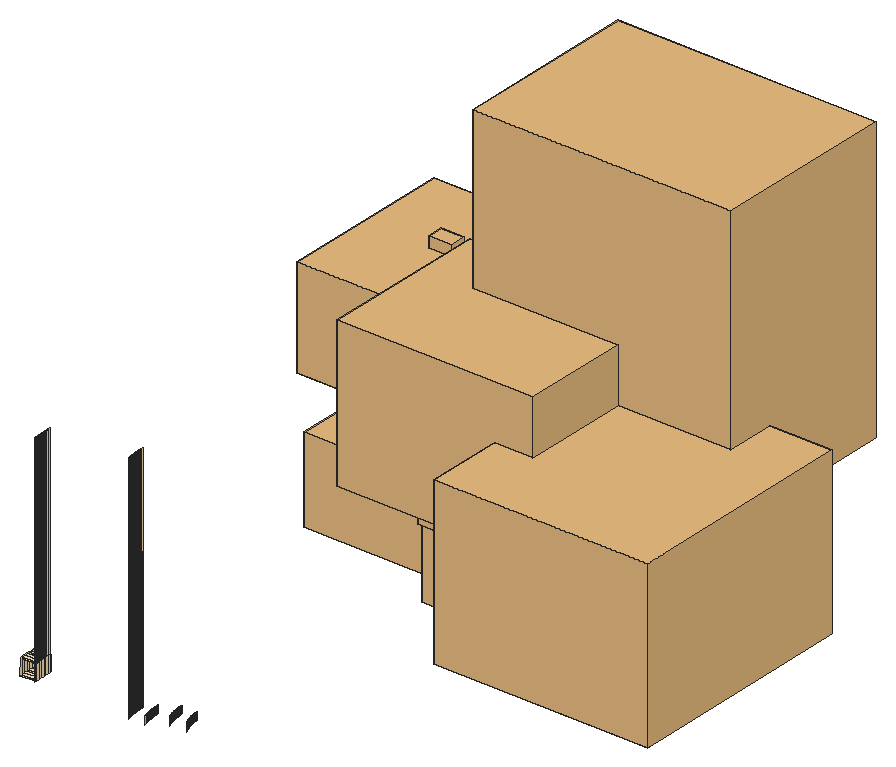
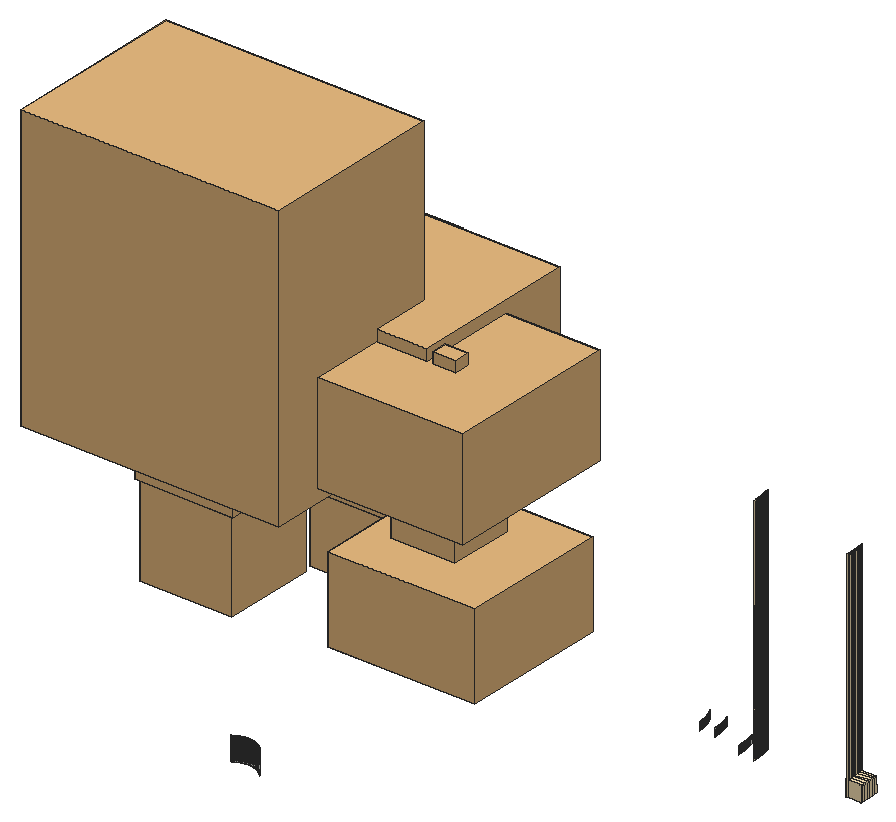
# SketchUp Ruby script. Lengths in inches.
U = 1.inch
M = Sketchup.active_model
def pt(a) = Geom::Point3d.new(a.map { |v| v * U })
def face(e, loops, mat)
  f = e.add_face(loops[0].map { |a| pt(a) })
  loops[1..].each { |l| e.add_face(l.map { |a| pt(a) }).erase! }
  f.material = f.back_material = mat if mat
  f
end
# faces: each face lists its corners as indices into pts; further lists are holes
def faces(e, pts, list, mat = nil) = list.each { |f| face(e, (f[0].is_a?(Array) ? f : [f]).map { |l| l.map { |i| pts[i] } }, mat) }
# xy, xz, yz: faces in a plane at the given z, y or x. An outline is a flat list of corners, or four numbers for a rectangle; further outlines are holes
def ring(l) = l.size == 4 ? [[l[0], l[1]], [l[2], l[1]], [l[2], l[3]], [l[0], l[3]]] : l.each_slice(2).to_a
def flat(e, list, mat, &to3) = list.each { |f| face(e, (f[0].is_a?(Array) ? f : [f]).map { |l| ring(l).map { |u, v| to3.(u, v) } }, mat) }
def xy(e, z, list, mat = nil) = flat(e, list, mat) { |x, y| [x, y, z] }
def xz(e, y, list, mat = nil) = flat(e, list, mat) { |x, z| [x, y, z] }
def yz(e, x, list, mat = nil) = flat(e, list, mat) { |y, z| [x, y, z] }
def lines(e, pts, list) = list.each { |a, b| e.add_line(pt(pts[a]), pt(pts[b])) }
# prism: a flat outline (further loops are holes) pulled along v
def prism(e, loops, v, mat = nil)
  f = face(e, loops, mat); d = Geom::Vector3d.new(v.map { |x| x * U })
  f.pushpull(f.normal.samedirection?(d) ? d.length : -d.length)
end
def box(e, o, s, mat = nil) = prism(e, [[o, [o[0] + s[0], o[1], o[2]], [o[0] + s[0], o[1] + s[1], o[2]], [o[0], o[1] + s[1], o[2]]]], [0, 0, s[2]], mat)
def at(x, y, z, deg = 0) = Geom::Transformation.translation(pt([x, y, z])) * Geom::Transformation.rotation(ORIGIN, Z_AXIS, deg.degrees)
def axes(o, x, y, z) = Geom::Transformation.new([*x, 0, *y, 0, *z, 0, *pt(o).to_a, 1])
def part(name) = M.definitions.add(name)
# library, detail: a bought-in or finely detailed component or shape, given as its bounding box
def library(name, o, s) = part(name).tap { |d| box(d.entities, o, s) }
def detail(e, o, s) = box(e.add_group.entities, o, s)
def put(e, d, t, mat = nil) = e.add_instance(d, t).tap { |i| i.material = mat if mat }
def group(e, t, mat = nil) = e.add_group.tap { |g| g.transformation = t; g.material = mat if mat }.entities
root = M.entities
M.materials.add("1026 AP 7946 SUNNY SIDE UP").color = [254, 231, 186]
M.materials.add("Material__10").color = [79, 108, 5]
M.materials.add("Material__5").color = [95, 70, 46]
M.materials.add("Material__6").color = [150, 168, 104]
M.materials.add("Material__7").color = [234, 233, 231]
M.materials.add("Material__8").color = [36, 36, 36]
M.materials.add("Material__9").color = [151, 172, 33]
M.materials.add("wire_1").color = [140, 184, 58]
M.materials.add("wire_2").color = [244, 244, 244]
M.materials.add("wire_4").color = [86, 225, 198]
M.materials.add("wire_5").color = [232, 232, 232]
c1 = library("Group\#97",[-915.9375,-34.5,735.6],[41.04,40.85,6.81])
c2 = library("Group\#96",[-991.92,-34.05,729.49],[10.64,7.28,57.53])
c3 = library("Group\#95",[-1022.2,-71.69,736.68],[86.94,78.77,45.64])
c4 = library("Group\#94",[-877.77,-100.41,669.81],[37.9,37.9,42.75])
c5 = library("Group\#93",[-957.79,-83.08,701.98],[44.29,44.29,27.78])
c6 = library("Group\#92",[-1023.9,-65.47,669.625],[67.53,67.55,39.17])
c7 = library("Group\#91",[-997.48,-49.45,708.79],[29.81,29.81,30.61])
c8 = library("Group\#90",[-956738.95,-82059.81,669752.625],[42194.58,42232.57,49521.48])
c9 = library("Group\#89",[-917.52,-36.6875,711.84],[44.99,44.98,28.22])
c10 = library("Group\#88",[-916244.63,-35413.97,669800.48],[42442.38,42642.99,59706.29])
c11 = library("Group\#87",[-955.48,-54.29,730.4],[118.63,83.7,130.4])
c12 = library("Group\#86",[-899.97,-18.72,732.17],[8.78,8.27,28.64])
c13 = library("Group\#85",[-906.16,-138.28,686.8],[98.25,106.18,75.79])
c14 = library("Group\#80",[-978.71,-103.24,719.12],[90.2,76.4,68.29])
c15 = library("Group\#75",[-955.98,-81.17,725.57],[41.03,40.85,6.81])
c16 = library("Group\#73",[-996.8,-48.73,736.67],[28.51,28.38,4.73])
c17 = library("Group\#72",[-876.58,-99.29,706.19],[35.74,35.58,5.93])
c18 = library("Group\#69",[-912.1,-32.49,735.82],[33.14,36.63,9.55])
c19 = library("Group\#68",[-994.36,-46.95,735.88],[24.38,25.9,6.88])
c20 = part("PLANT-30")
p = [[0,0,0],[1,0,0],[1,1,0]]
lines(c20.entities,p,[[0,1],[1,2],[2,0]])
put(c20.entities,c1,at(895.63,-7.06,-669.82),"Material__5")
put(c20.entities,c2,at(895.63,-7.06,-669.82),"wire_1")
put(c20.entities,c3,at(895.63,-7.06,-669.82),"Material__6")
put(c20.entities,c4,at(895.63,-7.06,-669.82),"wire_2")
put(c20.entities,c5,at(895.63,-7.06,-669.82),"wire_2")
put(c20.entities,c6,at(895.63,-7.06,-669.82),"Material__7")
put(c20.entities,c7,at(895.63,-7.06,-669.82),"wire_2")
put(c20.entities,c8,axes([895.63,-7.06,-669.82],[0.001,0,0],[0,0.001,0],[0,0,0.001]),"Material__8")
put(c20.entities,c9,at(895.63,-7.06,-669.82),"wire_2")
put(c20.entities,c10,axes([895.63,-7.06,-669.82],[0.001,0,0],[0,0.001,0],[0,0,0.001]),"Material__8")
put(c20.entities,c11,at(895.63,-7.06,-669.82),"Material__9")
put(c20.entities,c12,at(895.63,-7.06,-669.82),"wire_4")
put(c20.entities,c13,at(895.63,-7.06,-669.82),"Material__10")
put(c20.entities,c14,at(895.63,-7.06,-669.82),"Material__8")
put(c20.entities,c15,at(895.63,-7.06,-669.82),"Material__5")
put(c20.entities,c16,at(895.63,-7.06,-669.82),"Material__5")
put(c20.entities,c17,at(895.63,-7.06,-669.82),"Material__5")
put(c20.entities,c18,at(895.63,-7.06,-669.82),"wire_5")
put(c20.entities,c19,at(895.63,-7.06,-669.82),"wire_5")
xy(root,246,[[4.282,236.454,4.257,236.723,6.094,236.878,6.101,236.806,6.107,236.741,6.111,236.697,6.116,236.648,6.117,236.635],[6.117,236.635,6.116,236.648,6.111,236.697,6.107,236.741,6.101,236.806,6.094,236.878,6.25,236.891,6.272,236.65],[4.257,236.723,4.223,237.164,6.061,237.29,6.064,237.242,6.069,237.184,6.074,237.117,6.08,237.05,6.084,236.992,6.089,236.94,6.094,236.882,6.094,236.878],[6.094,236.878,6.094,236.882,6.089,236.94,6.084,236.992,6.08,237.05,6.074,237.117,6.069,237.184,6.064,237.242,6.061,237.29,6.218,237.301,6.25,236.891],[4.223,237.164,4.193,237.665,6.032,237.76,6.033,237.744,6.037,237.673,6.042,237.587,6.045,237.538,6.047,237.493,6.052,237.428,6.057,237.352,6.061,237.294,6.061,237.29],
  [6.061,237.29,6.061,237.294,6.057,237.352,6.052,237.428,6.047,237.493,6.045,237.538,6.042,237.587,6.037,237.673,6.033,237.744,6.032,237.76,6.191,237.768,6.218,237.301],[4.193,237.665,4.182,237.928,6.021,237.995,6.025,237.918,6.029,237.822,6.031,237.781,6.032,237.76],[6.032,237.76,6.031,237.781,6.029,237.822,6.025,237.918,6.021,237.995,6.18,238.001,6.191,237.768],[4.182,237.928,4.167,238.426,6.006,238.466,6.007,238.416,6.01,238.293,6.011,238.269,6.012,238.246,6.015,238.165,6.019,238.058,6.02,238.025,6.021,237.995],[6.021,237.995,6.02,238.025,6.019,238.058,6.015,238.165,6.012,238.246,6.011,238.269,6.01,238.293,6.007,238.416,6.006,238.466,6.167,238.47,6.18,238.001],
  [4.167,238.426,4.162,238.773,6.001,238.79,6.001,238.749,6.002,238.675,6.005,238.529,6.005,238.497,6.006,238.466],[6.006,238.466,6.005,238.497,6.005,238.529,6.002,238.675,6.001,238.749,6.001,238.79,6.162,238.792,6.167,238.47],[4.162,238.773,4.161,238.899,6,238.893,6,238.853,6.001,238.79],[6.001,238.79,6,238.853,6,238.893,6.161,238.893,6.162,238.792],[6,238.893,4.161,238.899,4.162,238.944,6,238.9375],
  [6,238.893,6,238.9375,6.162,238.937,6.161,238.893],[6,238.9375,4.162,238.944,4.162,238.948]],"1026 AP 7946 SUNNY SIDE UP")
xy(root,248,[[4.282,236.455,6.272,236.65,6.25,236.891,4.257,236.723],[4.257,236.723,6.25,236.891,6.218,237.301,4.223,237.164],[4.223,237.164,6.218,237.301,6.191,237.768,4.193,237.665],[4.193,237.665,6.191,237.768,6.18,238.001,6.021,237.995,4.182,237.928],[4.182,237.928,6.021,237.995,6.18,238.001,6.167,238.47,4.167,238.426],
  [4.167,238.426,6.167,238.47,6.162,238.792,4.162,238.773],[4.162,238.773,6.162,238.792,6.162,238.893,4.162,238.899],[6.162,238.893,6.162,238.937,4.162,238.944,4.162,238.899],[6.162,238.937,4.162,238.948,4.162,238.944]],"1026 AP 7946 SUNNY SIDE UP")
yz(root,4.162,[[238.944,246,238.948,248]],"1026 AP 7946 SUNNY SIDE UP")
yz(root,6.001,[[238.749,246,238.756,274],[238.756,246,238.764,274]],"1026 AP 7946 SUNNY SIDE UP")
yz(root,6.005,[[238.497,246,238.513,274],[238.513,246,238.529,274]],"1026 AP 7946 SUNNY SIDE UP")
yz(root,25,[[238.935,247,239,248]])
p = [[6.136,236.454,246],[6.14,236.413,246],[6.14,236.413,274],[6.136,236.454,274],[18.296,236.352,252],[18.262,236.505,252],
  [18.262,236.505,246],[18.296,236.352,246],[18.289,236.382,246],[18.262,236.505,246],[18.262,236.505,276],[18.289,236.382,276],
  [20.341,236.412,246],[20.308,236.538,246],[20.308,236.538,247],[20.341,236.412,247],[4.282,236.454,246],[4.282,236.455,248],
  [4.257,236.723,248],[4.257,236.723,246],[6.124,236.5625,246],[6.131,236.491,246],[6.131,236.491,274],[6.124,236.5625,274],
  [18.231,236.659,252],[18.231,236.659,246],[18.237,236.628,246],[18.237,236.628,276],[20.276,236.666,246],[20.276,236.666,247],
  [6.111,236.697,246],[6.116,236.648,246],[6.116,236.648,274],[6.111,236.697,274],[6.117,236.635,246],[18.213,236.751,246],
  [18.213,236.751,276],[4.223,237.164,248],[4.223,237.164,246],[6.101,236.806,246],[6.107,236.741,246],[6.107,236.741,274],
  [6.101,236.806,274],[6.272,236.65,248],[6.272,236.65,246],[6.25,236.891,246],[6.25,236.891,248],[18.201,236.813,252],
  [18.201,236.813,246],[20.247,236.793,246],[20.247,236.793,247],[6.094,236.882,246],[6.094,236.878,246],[6.094,236.882,274],
  [18.173,236.968,252],[18.173,236.968,246],[18.19,236.875,246],[18.19,236.875,276],[20.219,236.921,246],[20.219,236.921,247],
  [6.084,236.992,246],[6.089,236.94,246],[6.089,236.94,274],[6.084,236.992,274],[6.218,237.301,246],[6.218,237.301,248],
  [18.168,236.999,246],[18.168,236.999,276],[20.192,237.049,246],[20.192,237.049,247],[6.08,237.05,246],[6.08,237.05,274],
  [18.148,237.123,252],[18.148,237.123,246],[18.148,237.123,246],[18.148,237.123,276],[20.167,237.178,246],[20.167,237.178,247],
  [6.069,237.184,246],[6.074,237.117,246],[6.074,237.117,274],[6.069,237.184,274],[18.124,237.278,252],[18.124,237.278,246],
  [18.129,237.247,246],[18.129,237.247,276],[4.193,237.665,248],[4.193,237.665,246],[6.061,237.294,246],[6.061,237.29,246],
  [6.064,237.242,246],[6.064,237.242,274],[6.061,237.294,274],[18.111,237.371,246],[18.111,237.371,276],[20.144,237.307,246],
  [20.144,237.307,247],[6.057,237.352,246],[6.057,237.352,274],[6.191,237.768,246],[6.191,237.768,248],[18.103,237.434,252],
  [18.103,237.434,246],[20.123,237.436,246],[20.123,237.436,247],[6.047,237.493,246],[6.052,237.428,246],[6.052,237.428,274],
  [6.047,237.493,274],[18.083,237.59,252],[18.083,237.59,246],[18.095,237.496,246],[18.095,237.496,276],[20.103,237.565,246],
  [20.103,237.565,247],[6.042,237.587,246],[6.045,237.538,246],[6.045,237.538,274],[6.042,237.587,274],[18.08,237.621,246],
  [18.08,237.621,276],[6.037,237.673,246],[6.037,237.673,274],[18.066,237.746,252],[18.066,237.746,246],[18.066,237.746,246],
  [18.066,237.746,276],[20.086,237.695,246],[20.086,237.695,247],[4.182,237.928,248],[4.182,237.928,246],[6.031,237.781,246],
  [6.032,237.76,246],[6.033,237.744,246],[6.033,237.744,274],[6.031,237.781,274],[18.05,237.902,252],[18.05,237.902,246],
  [18.053,237.871,246],[18.053,237.871,276],[20.069,237.825,246],[20.069,237.825,247],[6.025,237.918,246],[6.029,237.822,246],
  [6.029,237.822,274],[6.025,237.918,274],[6.18,238.001,246],[6.18,238.001,248],[20.055,237.955,246],[20.055,237.955,247],
  [4.167,238.426,248],[4.167,238.426,246],[6.021,237.995,246],[6.021,237.995,274],[6.021,237.995,248],[18.037,238.058,252],
  [18.037,238.058,246],[18.042,237.996,246],[18.042,237.996,276],[6.019,238.058,246],[6.02,238.025,246],[6.02,238.025,274],
  [6.019,238.058,274],[6.167,238.47,246],[6.167,238.47,248],[18.032,238.121,246],[18.032,238.121,276],[20.042,238.085,246],
  [20.042,238.085,247],[6.015,238.165,246],[6.015,238.165,274],[18.026,238.215,252],[18.026,238.215,246],[18.024,238.247,246],
  [18.024,238.247,276],[20.031,238.215,246],[20.031,238.215,247],[6.011,238.269,246],[6.012,238.246,246],[6.012,238.246,274],
  [6.011,238.269,274],[18.016,238.372,252],[18.016,238.372,246],[18.016,238.372,246],[18.016,238.372,276],[20.021,238.346,246],
  [20.021,238.346,247],[6.007,238.416,246],[6.01,238.293,246],[6.01,238.293,274],[6.007,238.416,274],[20.014,238.477,246],
  [20.014,238.477,247],[4.162,238.773,248],[4.162,238.773,246],[6.005,238.497,246],[6.006,238.466,246],[6.005,238.497,274],
  [18.009,238.529,252],[18.009,238.529,246],[18.011,238.497,246],[18.011,238.497,276],[6.002,238.675,246],[6.005,238.529,246],
  [6.005,238.529,274],[6.002,238.675,274],[6.162,238.792,246],[6.162,238.792,248],[18.004,238.686,252],[18.004,238.686,246],
  [18.006,238.623,246],[18.006,238.623,276],[20.008,238.607,246],[20.008,238.607,247],[18.003,238.749,246],[18.003,238.749,276],
  [20.003,238.738,246],[20.003,238.738,247],[6.001,238.749,246],[6.001,238.749,274],[18.001,238.843,252],[18.001,238.843,246],
  [18,238.872,246],[18,239,246],[18,239,276],[20.001,238.869,246],[20.001,238.869,247],[4.162,238.899,248],
  [4.161,238.899,246],[6.001,238.764,246],[6.001,238.764,274],[6,239,274],[6,239,248],[6,239,246],
  [5.999,238.956,246],[6,238.9375,246],[6,238.893,246],[6,238.853,246],[6.001,238.79,246],[6.161,238.893,246],
  [6.162,238.893,248],[18,239,252],[18,239,246],[4.162,238.944,248],[4.162,238.944,246],[6.162,238.937,248],
  [4.162,238.948,248],[4.162,238.948,246],[6.162,238.937,246],[20,239,246],[20,239,247],[23.498,236.406,248],
  [23.498,236.406,247],[23.465,236.491,247],[23.465,236.491,248],[25.67,236.5,247],[25.703,236.444,247],[25.703,236.444,248],
  [25.67,236.5,248],[23.433,236.577,247],[23.433,236.577,248],[25.638,236.557,247],[25.638,236.557,248],[23.402,236.663,247],
  [23.402,236.663,248],[25.575,236.672,247],[25.606,236.614,247],[25.606,236.614,248],[25.575,236.672,248],[23.371,236.75,248],
  [23.371,236.75,247],[23.343,236.837,247],[23.343,236.837,248],[25.516,236.789,247],[25.545,236.73,247],[25.545,236.73,248],
  [25.516,236.789,248],[23.315,236.924,247],[23.315,236.924,248],[25.459,236.907,247],[25.487,236.847,247],[25.487,236.847,248],
  [25.459,236.907,248],[23.288,237.012,247],[23.288,237.012,248],[25.432,236.966,247],[25.432,236.966,248],[23.263,237.1,247],
  [23.263,237.1,248],[25.381,237.087,247],[25.406,237.026,247],[25.406,237.026,248],[25.381,237.087,248],[23.239,237.188,247],
  [23.239,237.188,248],[25.332,237.208,247],[25.356,237.147,247],[25.356,237.147,248],[25.332,237.208,248],[23.215,237.277,247],
  [23.215,237.277,248],[25.309,237.269,247],[25.309,237.269,248],[23.193,237.366,247],[23.193,237.366,248],[25.265,237.393,247],
  [25.287,237.331,247],[25.287,237.331,248],[25.265,237.393,248],[23.173,237.455,247],[23.173,237.455,248],[25.245,237.455,247],
  [25.245,237.455,248],[23.153,237.545,248],[23.153,237.545,247],[23.135,237.634,247],[23.135,237.634,248],[25.206,237.58,247],
  [25.225,237.517,247],[25.225,237.517,248],[25.206,237.58,248],[23.117,237.724,247],[23.117,237.724,248],[25.17,237.706,247],
  [25.188,237.643,247],[25.188,237.643,248],[25.17,237.706,248],[23.101,237.815,247],[23.101,237.815,248],[25.154,237.769,247],
  [25.154,237.769,248],[23.086,237.905,247],[23.086,237.905,248],[25.123,237.897,247],[25.138,237.833,247],[25.138,237.833,248],
  [25.123,237.897,248],[23.072,237.996,247],[23.072,237.996,248],[25.109,237.96,247],[25.109,237.96,248],[23.06,238.086,247],
  [23.06,238.086,248],[25.084,238.089,247],[25.096,238.025,247],[25.096,238.025,248],[25.084,238.089,248],[23.049,238.177,247],
  [23.049,238.177,248],[25.072,238.153,247],[25.072,238.153,248],[23.038,238.268,247],[23.038,238.268,248],[25.052,238.283,247],
  [25.062,238.218,247],[25.062,238.218,248],[25.052,238.283,248],[23.029,238.359,247],[23.029,238.359,248],[25.035,238.412,247],
  [25.043,238.347,247],[25.043,238.347,248],[25.035,238.412,248],[23.022,238.451,247],[23.022,238.451,248],[25.027,238.477,247],
  [25.027,238.477,248],[23.015,238.542,248],[23.015,238.542,247],[23.01,238.634,247],[23.01,238.634,248],[25.015,238.608,247],
  [25.021,238.542,247],[25.021,238.542,248],[25.015,238.608,248],[23.005,238.725,247],[23.005,238.725,248],[25.011,238.673,247],
  [25.011,238.673,248],[23.002,238.817,247],[23.002,238.817,248],[25.004,238.804,247],[25.007,238.738,247],[25.007,238.738,248],
  [25.004,238.804,248],[23.001,238.908,247],[23.001,238.908,248],[25.002,238.869,247],[25.002,238.869,248],[23,239,247],
  [23,239,248],[25,238.935,247],[25,238.935,248],[55.354,272.833,250],[55.354,272.833,247],[55.278,272.852,247],
  [55.278,272.852,250],[55.431,272.816,250],[55.431,272.816,247],[55.508,272.8,250],[55.508,272.8,247],[55.585,272.787,250],
  [55.585,272.787,247],[55.663,272.776,250],[55.663,272.776,247],[55.741,272.766,250],[55.741,272.766,247],[55.819,272.759,250],
  [55.819,272.759,247],[55.898,272.754,250],[55.898,272.754,247],[55.976,272.751,250],[55.976,272.751,247],[56.055,272.75,250],
  [56.055,272.75,247],[56.133,272.751,250],[56.133,272.751,247],[56.212,272.754,250],[56.212,272.754,247],[56.29,272.759,250],
  [56.29,272.759,247],[56.368,272.766,250],[56.368,272.766,247],[56.446,272.776,250],[56.446,272.776,247],[56.524,272.787,250],
  [56.524,272.787,247],[56.601,272.8,250],[56.601,272.8,247],[56.679,272.816,250],[56.679,272.816,247],[56.755,272.833,250],
  [56.755,272.833,247],[56.831,272.852,250],[56.831,272.852,247],[54.98,272.949,250],[54.98,272.949,247],[54.907,272.978,247],
  [54.907,272.978,250],[55.053,272.922,250],[55.053,272.922,247],[55.128,272.897,250],[55.128,272.897,247],[55.203,272.874,250],
  [55.203,272.874,247],[56.907,272.874,250],[56.907,272.874,247],[56.982,272.897,250],[56.982,272.897,247],[57.056,272.922,250],
  [57.056,272.922,247],[57.13,272.949,250],[57.13,272.949,247],[57.203,272.978,250],[57.203,272.978,247],[54.763,273.042,250],
  [54.763,273.042,247],[54.693,273.077,247],[54.693,273.077,250],[54.835,273.009,250],[54.835,273.009,247],[57.275,273.009,250],
  [57.275,273.009,247],[57.346,273.042,250],[57.346,273.042,247],[57.417,273.077,250],[57.417,273.077,247],[54.623,273.114,250],
  [54.623,273.114,247],[54.555,273.152,247],[54.555,273.152,250],[57.486,273.114,250],[57.486,273.114,247],[57.555,273.152,250],
  [57.555,273.152,247],[54.421,273.234,250],[54.421,273.234,247],[54.356,273.278,247],[54.356,273.278,250],[54.487,273.192,250],
  [54.487,273.192,247],[57.622,273.192,250],[57.622,273.192,247],[57.689,273.234,250],[57.689,273.234,247],[57.754,273.278,250],
  [57.754,273.278,247],[54.291,273.323,250],[54.291,273.323,247],[54.228,273.37,247],[54.228,273.37,250],[57.818,273.323,250],
  [57.818,273.323,247],[57.881,273.37,250],[57.881,273.37,247],[54.167,273.419,250],[54.167,273.419,247],[54.106,273.469,247],
  [54.106,273.469,250],[54.047,273.521,250],[54.047,273.521,247],[53.99,273.574,247],[53.99,273.574,250],[53.933,273.629,250],
  [53.933,273.629,247],[53.879,273.685,247],[53.879,273.685,250],[53.825,273.743,250],[53.825,273.743,247],[53.774,273.802,247],
  [53.774,273.802,250],[53.723,273.862,247],[53.723,273.862,250],[18.262,236.505,264],[18.231,236.659,264],[18.231,236.659,252],
  [18.262,236.505,252],[18.201,236.813,264],[18.201,236.813,252],[18.173,236.968,264],[18.173,236.968,252],[18.148,237.123,264],
  [18.148,237.123,252],[18.124,237.278,264],[18.124,237.278,252],[18.103,237.434,264],[18.103,237.434,252],[18.083,237.59,264],
  [18.083,237.59,252],[18.066,237.746,264],[18.066,237.746,252],[18.05,237.902,264],[18.05,237.902,252],[18.037,238.058,264],
  [18.037,238.058,252],[18.026,238.215,264],[18.026,238.215,252],[18.016,238.372,264],[18.016,238.372,252],[18.009,238.529,264],
  [18.009,238.529,252],[18.004,238.686,264],[18.004,238.686,252],[18.001,238.843,264],[18.001,238.843,252],[18,239,264],
  [18,239,252]]
faces(root,p,[[0,1,2,3],[8,9,10,11],[16,17,18,19],[20,21,22,23],[21,0,3,22],[9,26,27,10],[30,31,32,33],[31,34,20,23,32],
  [26,35,36,27],[19,18,37,38],[39,40,41,42],[40,30,33,41],[43,44,45,46],[51,52,39,42,53],[35,56,57,36],[60,61,62,63],
  [61,51,53,62],[46,45,64,65],[56,66,67,57],[70,60,63,71],[66,74,75,67],[78,79,80,81],[79,70,71,80],[74,84,85,75],
  [38,37,86,87],[88,89,90,91,92],[90,78,81,91],[84,93,94,85],[97,88,92,98],[65,64,99,100],[105,106,107,108],[106,97,98,107],
  [93,111,112,94],[115,116,117,118],[116,105,108,117],[111,119,120,112],[121,115,118,122],[119,125,126,120],[87,86,129,130],[131,132,133,134,135],
  [133,121,122,134],[125,138,139,126],[142,143,144,145],[143,131,135,144],[100,99,146,147],[130,129,150,151],[152,142,145,153,154],[138,157,158,139],
  [159,160,161,162],[160,152,154,153,161],[147,146,163,164],[157,165,166,158],[169,159,162,170],[165,173,174,166],[177,178,179,180],[178,169,170,179],
  [173,183,184,174],[187,188,189,190],[188,177,180,189],[151,150,193,194],[195,196,187,190,197],[183,200,201,184],[202,203,204,205],[164,163,206,207],
  [200,210,211,201],[210,214,215,211],[218,202,205,219],[222,223,224,215,214],[194,193,227,228],[229,230,231,232,233,234,235,236,237,238],[207,206,239,240],[227,243,244,228],
  [245,246,247,235,248],[248,245,240,239]],"1026 AP 7946 SUNNY SIDE UP")
faces(root,p,[[4,5,6,7],[12,13,14,15],[5,24,25,6],[13,28,29,14],[24,47,48,25],[28,49,50,29],[47,54,55,48],[49,58,59,50],
  [58,68,69,59],[54,72,73,55],[68,76,77,69],[72,82,83,73],[76,95,96,77],[82,101,102,83],[95,103,104,96],[101,109,110,102],
  [103,113,114,104],[109,123,124,110],[113,127,128,114],[123,136,137,124],[127,140,141,128],[140,148,149,141],[136,155,156,137],[148,167,168,149],
  [155,171,172,156],[167,175,176,168],[171,181,182,172],[175,185,186,176],[185,191,192,186],[181,198,199,182],[198,208,209,199],[191,212,213,192],
  [212,216,217,213],[208,220,221,209],[216,225,226,217],[220,241,242,221],[225,249,250,226],[251,252,253,254],[255,256,257,258],[254,253,259,260],
  [261,255,258,262],[260,259,263,264],[265,266,267,268],[266,261,262,267],[269,270,271,272],[264,263,270,269],[273,274,275,276],[274,265,268,275],
  [272,271,277,278],[279,280,281,282],[280,273,276,281],[278,277,283,284],[285,279,282,286],[284,283,287,288],[289,290,291,292],[290,285,286,291],
  [288,287,293,294],[295,296,297,298],[296,289,292,297],[294,293,299,300],[301,295,298,302],[300,299,303,304],[305,306,307,308],[306,301,302,307],
  [304,303,309,310],[311,305,308,312],[313,314,315,316],[310,309,314,313],[317,318,319,320],[318,311,312,319],[316,315,321,322],[323,324,325,326],
  [324,317,320,325],[322,321,327,328],[329,323,326,330],[328,327,331,332],[333,334,335,336],[334,329,330,335],[332,331,337,338],[339,333,336,340],
  [338,337,341,342],[343,344,345,346],[344,339,340,345],[342,341,347,348],[349,343,346,350],[348,347,351,352],[353,354,355,356],[354,349,350,355],
  [352,351,357,358],[359,360,361,362],[360,353,356,361],[358,357,363,364],[365,359,362,366],[367,368,369,370],[364,363,368,367],[371,372,373,374],
  [372,365,366,373],[370,369,375,376],[377,371,374,378],[376,375,379,380],[381,382,383,384],[382,377,378,383],[380,379,385,386],[387,381,384,388],
  [386,385,389,390],[391,387,388,392],[393,394,395,396],[397,398,394,393],[399,400,398,397],[401,402,400,399],[403,404,402,401],[405,406,404,403],
  [407,408,406,405],[409,410,408,407],[411,412,410,409],[413,414,412,411],[415,416,414,413],[417,418,416,415],[419,420,418,417],[421,422,420,419],
  [423,424,422,421],[425,426,424,423],[427,428,426,425],[429,430,428,427],[431,432,430,429],[433,434,432,431],[435,436,437,438],[439,440,436,435],
  [441,442,440,439],[443,444,442,441],[396,395,444,443],[445,446,434,433],[447,448,446,445],[449,450,448,447],[451,452,450,449],[453,454,452,451],
  [455,456,457,458],[459,460,456,455],[438,437,460,459],[461,462,454,453],[463,464,462,461],[465,466,464,463],[467,468,469,470],[458,457,468,467],
  [471,472,466,465],[473,474,472,471],[475,476,477,478],[479,480,476,475],[470,469,480,479],[481,482,474,473],[483,484,482,481],[485,486,484,483],
  [487,488,489,490],[478,477,488,487],[491,492,486,485],[493,494,492,491],[495,496,497,498],[490,489,496,495],[499,500,501,502],[498,497,500,499],
  [503,504,505,506],[502,501,504,503],[507,508,509,510],[506,505,508,507],[510,509,511,512],[513,514,515,516],[514,517,518,515],[517,519,520,518],
  [519,521,522,520],[521,523,524,522],[523,525,526,524],[525,527,528,526],[527,529,530,528],[529,531,532,530],[531,533,534,532],[533,535,536,534],
  [535,537,538,536],[537,539,540,538],[539,541,542,540],[541,543,544,542],[543,545,546,544]])
put(root,c20,axes([63.27,273.59,263.86],[0.28,0,0],[0,0.28,0],[0,0,0.28]),"1026 AP 7946 SUNNY SIDE UP")
